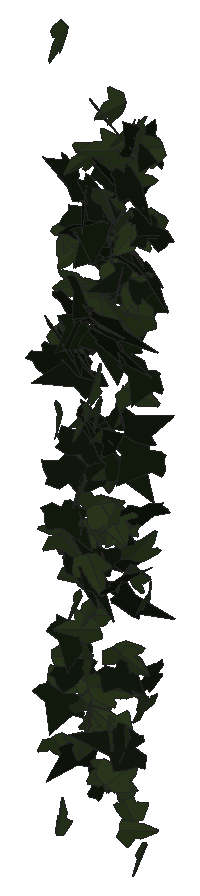
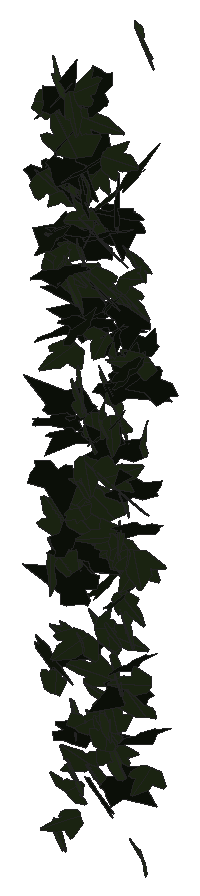
# SketchUp Ruby script. Lengths in inches.
U = 1.inch
M = Sketchup.active_model
def pt(a) = Geom::Point3d.new(a.map { |v| v * U })
def face(e, loops, mat)
  f = e.add_face(loops[0].map { |a| pt(a) })
  loops[1..].each { |l| e.add_face(l.map { |a| pt(a) }).erase! }
  f.material = f.back_material = mat if mat
  f
end
# faces: each face lists its corners as indices into pts; further lists are holes
def faces(e, pts, list, mat = nil) = list.each { |f| face(e, (f[0].is_a?(Array) ? f : [f]).map { |l| l.map { |i| pts[i] } }, mat) }
# xy, xz, yz: faces in a plane at the given z, y or x. An outline is a flat list of corners, or four numbers for a rectangle; further outlines are holes
def ring(l) = l.size == 4 ? [[l[0], l[1]], [l[2], l[1]], [l[2], l[3]], [l[0], l[3]]] : l.each_slice(2).to_a
def flat(e, list, mat, &to3) = list.each { |f| face(e, (f[0].is_a?(Array) ? f : [f]).map { |l| ring(l).map { |u, v| to3.(u, v) } }, mat) }
def xy(e, z, list, mat = nil) = flat(e, list, mat) { |x, y| [x, y, z] }
def xz(e, y, list, mat = nil) = flat(e, list, mat) { |x, z| [x, y, z] }
def yz(e, x, list, mat = nil) = flat(e, list, mat) { |y, z| [x, y, z] }
def lines(e, pts, list) = list.each { |a, b| e.add_line(pt(pts[a]), pt(pts[b])) }
# prism: a flat outline (further loops are holes) pulled along v
def prism(e, loops, v, mat = nil)
  f = face(e, loops, mat); d = Geom::Vector3d.new(v.map { |x| x * U })
  f.pushpull(f.normal.samedirection?(d) ? d.length : -d.length)
end
def box(e, o, s, mat = nil) = prism(e, [[o, [o[0] + s[0], o[1], o[2]], [o[0] + s[0], o[1] + s[1], o[2]], [o[0], o[1] + s[1], o[2]]]], [0, 0, s[2]], mat)
def at(x, y, z, deg = 0) = Geom::Transformation.translation(pt([x, y, z])) * Geom::Transformation.rotation(ORIGIN, Z_AXIS, deg.degrees)
def axes(o, x, y, z) = Geom::Transformation.new([*x, 0, *y, 0, *z, 0, *pt(o).to_a, 1])
def part(name) = M.definitions.add(name)
# library, detail: a bought-in or finely detailed component or shape, given as its bounding box
def library(name, o, s) = part(name).tap { |d| box(d.entities, o, s) }
def detail(e, o, s) = box(e.add_group.entities, o, s)
def put(e, d, t, mat = nil) = e.add_instance(d, t).tap { |i| i.material = mat if mat }
def group(e, t, mat = nil) = e.add_group.tap { |g| g.transformation = t; g.material = mat if mat }.entities
root = M.entities
M.materials.add("1026 AP 7946 SUNNY SIDE UP").color = [254, 231, 186]
M.materials.add("efeu1").color = [18, 25, 13]
M.materials.add("efeu2").color = [43, 57, 29]
c1 = part("ivyleaf_10")
p = [[0,0.5,-0.03],[-0.0625,2.02,-0.43],[-0.19,2.01,-0.46],[-0.54,1.05,-0.29],[-0.52,0.625,-0.18],[-0.83,0.76,-0.28],
  [-1.16,0.64,-0.33],[-1.15,0.33,-0.24],[-0.77,-0.39,0.02],[-0.3,-0.51,0.16],[0.04,-0.48,0.23],[-0.02,2.01,-0.4375],
  [-0.06,2.01,-0.43],[0.04,-0.49,0.23],[0.67,-0.49,0.14],[1.38,0.36,-0.2],[1.375,0.51,-0.24],[0.81,0.65,-0.19],
  [0.62,0.59,-0.15],[0.6,1.09,-0.28],[0.5,1.23,-0.31]]
faces(c1.entities,p,[[0,1,2,3,4,5,6,7,8,9,10],[11,12,0,13,14,15,16,17,18,19,20]],"efeu2")
c2 = part("ivyleaf_9")
p = [[1.54,2.16,1.25],[1.36,2.04,1.19],[-0.21,0.99,0.68],[-0.71,1.11,0.82],[-0.85,0.86,0.67],[-0.8,0.17,0.21],
  [-0.9,-0.01,0.1],[-0.67,-0.16,-0.02],[-0.08,-0.08,-0.05],[-0.03,-0.6,-0.4],[0.65,-0.88,-0.66],[0.83,-0.6,-0.49],
  [1.29,-0.42,-0.43],[1.8125,-0.07,-0.26],[1.21,0.44,0.15]]
faces(c2.entities,p,[[0,1,2,3,4,5,6,7,8,9,10,11,12,13,14]],"efeu1")
put(root,c1,axes([111.04,211.59,258.61],[0.30252,-0.15607,0.01746],[0.00318,-0.02574,-0.25464],[0.24698,0.1915,-0.01812]),"1026 AP 7946 SUNNY SIDE UP")
put(root,c2,axes([110.8125,211.57,261.93],[0.31359,-0.0983,0.17351],[0.21726,-0.0999,-0.22844],[0.21747,0.24155,-0.02198]),"1026 AP 7946 SUNNY SIDE UP")
put(root,c2,axes([110.88,211.54,262.32],[0.30214,-0.05478,0.18215],[0.25651,-0.07125,-0.20544],[0.13851,0.25143,-0.01687]),"1026 AP 7946 SUNNY SIDE UP")
put(root,c2,axes([109.72,211.71,261.66],[0.07676,-0.16825,0.19826],[0.10699,-0.18132,-0.18125],[0.38863,0.08315,0.01074]),"1026 AP 7946 SUNNY SIDE UP")
put(root,c1,axes([110.43,211.59,260.29],[0.19919,-0.26197,-0.00928],[-0.01864,0.00261,-0.2996],[0.41167,0.12687,-0.00908]),"1026 AP 7946 SUNNY SIDE UP")
put(root,c1,axes([109.73,211.73,259.9375],[-0.01994,0.01186,0.27147],[0.24473,-0.21258,0.01633],[0.33474,0.15613,0.00423]),"1026 AP 7946 SUNNY SIDE UP")
put(root,c1,axes([110.51,211.61,257.3],[0.33232,0.00269,0.16449],[0.24963,-0.03192,-0.21614],[0.0269,0.26294,-0.02637]),"1026 AP 7946 SUNNY SIDE UP")
put(root,c1,axes([111.43,211.56,262.43],[-0.38192,0.01159,-0.18672],[-0.28045,0.04243,0.24918],[0.0544,0.30011,-0.02623]),"1026 AP 7946 SUNNY SIDE UP")
put(root,c1,axes([110.82,211.48,254.89],[-0.07067,-0.00583,0.26294],[0.34009,0.13688,0.04325],[-0.21338,0.2201,-0.01814]),"1026 AP 7946 SUNNY SIDE UP")
put(root,c1,axes([110.96,211.53,258.52],[0.32672,0.13462,0.13671],[0.18289,0.06295,-0.25451],[-0.23322,0.23795,-0.00807]),"1026 AP 7946 SUNNY SIDE UP")
put(root,c1,axes([111.46,211.49,254.04],[0.10164,-0.19933,-0.15373],[-0.05275,0.14462,-0.21476],[0.38688,0.07208,0.01111]),"1026 AP 7946 SUNNY SIDE UP")
put(root,c2,axes([110.3125,211.77,261.92],[-0.2114,-0.15335,0.13328],[-0.09465,-0.11882,-0.20882],[0.30187,-0.14464,0.02786]),"1026 AP 7946 SUNNY SIDE UP")
put(root,c2,axes([110.28,211.83,262.58],[-0.06592,-0.16503,0.247],[-0.05104,-0.23902,-0.17606],[0.45604,-0.05061,0.016]),"1026 AP 7946 SUNNY SIDE UP")
put(root,c1,axes([110.35,211.625,258.81],[0.14496,-0.22878,-0.01015],[-0.01654,0.00498,-0.25394],[0.3596,0.09245,-0.00759]),"1026 AP 7946 SUNNY SIDE UP")
put(root,c2,axes([109.92,211.6,258.18],[0.01376,-0.19547,-0.15045],[0.09737,0.14204,-0.19267],[0.37004,-0.03011,0.05629]),"1026 AP 7946 SUNNY SIDE UP")
put(root,c2,axes([110.08,211.77,264.91],[0.11972,-0.28684,-0.03214],[0.04752,-0.02247,0.30466],[-0.45093,-0.07852,0.02358]),"1026 AP 7946 SUNNY SIDE UP")
put(root,c1,axes([110.48,211.7,255.89],[-0.09368,-0.01887,0.24048],[-0.28086,-0.15228,-0.06051],[0.23841,-0.18681,0.02321]),"1026 AP 7946 SUNNY SIDE UP")
put(root,c2,axes([111.2,211.54,255.375],[0.00797,-0.13008,-0.21277],[0.01462,0.20579,-0.13257],[0.38253,-0.00515,0.0095]),"1026 AP 7946 SUNNY SIDE UP")
put(root,c1,axes([109.84,211.67,267.88],[0.26284,-0.25087,0.012],[-0.00612,-0.01829,-0.31036],[0.39496,0.16667,-0.01279]),"1026 AP 7946 SUNNY SIDE UP")
put(root,c1,axes([111.1875,211.7,257.14],[0.03813,-0.20313,-0.09742],[0.06358,-0.08842,0.20839],[-0.34575,-0.03866,0.02758]),"1026 AP 7946 SUNNY SIDE UP")
put(root,c2,axes([111.21,211.41,257.17],[-0.05601,0.19,-0.1722],[-0.03869,0.1665,0.20005],[0.39716,0.04302,-0.0048]),"1026 AP 7946 SUNNY SIDE UP")
put(root,c2,axes([111.38,211.77,253.75],[-0.15816,-0.15471,-0.22356],[-0.19168,-0.17849,0.18903],[-0.37139,0.15801,-0.00236]),"1026 AP 7946 SUNNY SIDE UP")
put(root,c2,axes([110.59,211.73,259.74],[-0.09981,-0.00293,0.27434],[0.25802,-0.21606,0.03657],[0.32984,0.16813,0.0544]),"1026 AP 7946 SUNNY SIDE UP")
put(root,c1,axes([110.45,211.6875,253.625],[-0.23115,-0.16581,0.07334],[-0.05359,-0.06589,-0.22797],[0.27923,-0.14991,0.01696]),"1026 AP 7946 SUNNY SIDE UP")
put(root,c1,axes([109.74,211.59,253.39],[-0.18971,-0.14311,-0.11144],[0.13133,0.06946,-0.19167],[0.24877,-0.1458,0.0162]),"1026 AP 7946 SUNNY SIDE UP")
put(root,c2,axes([111.46,211.82,263.36],[-0.01003,-0.07,-0.263],[-0.0769,-0.25025,0.0706],[-0.40846,0.04883,-0.00684]),"1026 AP 7946 SUNNY SIDE UP")
put(root,c1,axes([111.11,211.77,265.89],[-0.10047,-0.0406,0.28246],[-0.32021,-0.18435,-0.07803],[0.29619,-0.21307,0.01146]),"1026 AP 7946 SUNNY SIDE UP")
put(root,c2,axes([109.77,211.83,254.22],[-0.17093,-0.23263,0.05842],[-0.0224,-0.05733,-0.26461],[0.37633,-0.10907,0.01078]),"1026 AP 7946 SUNNY SIDE UP")
put(root,c1,axes([111.22,211.74,255.57],[-0.06018,-0.01159,-0.24218],[0.30076,-0.14021,-0.02579],[-0.21549,-0.19246,0.03164]),"1026 AP 7946 SUNNY SIDE UP")
put(root,c1,axes([111.1,211.53,253.09],[0.25615,0.08611,-0.18998],[0.22602,0.11942,0.18846],[0.22755,-0.21556,0.02666]),"1026 AP 7946 SUNNY SIDE UP")
put(root,c1,axes([111.26,211.73,264.59],[0.06491,-0.26607,0.03363],[0.00067,-0.03449,-0.27754],[0.4218,0.041,-0.00474]),"1026 AP 7946 SUNNY SIDE UP")
put(root,c2,axes([111.62,211.85,261.5],[-0.14273,-0.21925,0.09189],[-0.02525,-0.09094,-0.24423],[0.37207,-0.09028,0.01868]),"1026 AP 7946 SUNNY SIDE UP")
put(root,c2,axes([110.45,211.73,256.98],[0.18394,-0.23826,-0.02048],[-0.02931,0.01147,-0.27311],[0.37463,0.11788,-0.01131]),"1026 AP 7946 SUNNY SIDE UP")
put(root,c1,axes([110.81,211.69,264.87],[-0.34515,0.07392,-0.09062],[0.10977,-0.06595,-0.23583],[-0.14412,-0.22725,0.03739]),"1026 AP 7946 SUNNY SIDE UP")
put(root,c2,axes([110.23,211.88,261.85],[0.03763,-0.09908,-0.23194],[0.18695,-0.19273,0.09952],[-0.33767,-0.11774,0.02925]),"1026 AP 7946 SUNNY SIDE UP")
put(root,c1,axes([111.42,211.84,266.28],[0.08577,-0.18091,-0.2197],[0.13687,-0.1944,0.19262],[-0.41659,-0.10111,0.01805]),"1026 AP 7946 SUNNY SIDE UP")
put(root,c1,axes([111.4,211.79,264.29],[0.21146,0.13552,-0.16404],[-0.14874,-0.13043,-0.19648],[-0.29425,0.16332,-0.01857]),"1026 AP 7946 SUNNY SIDE UP")
put(root,c1,axes([109.84,211.65,254.59],[0.32946,-0.00035,-0.08441],[0.12818,0.02364,0.21478],[0.01302,-0.22373,0.0215]),"1026 AP 7946 SUNNY SIDE UP")
put(root,c1,axes([111.59,211.79,251.71],[0.15704,-0.1968,0.08996],[0.05404,-0.0817,-0.22775],[0.33493,0.10546,-0.00543]),"1026 AP 7946 SUNNY SIDE UP")
put(root,c2,axes([111.29,211.69,265.47],[0.18631,-0.24542,-0.14088],[-0.11516,0.11473,-0.27969],[0.42538,0.13855,-0.01402]),"1026 AP 7946 SUNNY SIDE UP")
put(root,c2,axes([110.43,211.79,264.25],[-0.19814,-0.22234,-0.08522],[0.07164,0.06779,-0.26282],[0.36538,-0.13387,0.00532]),"1026 AP 7946 SUNNY SIDE UP")
put(root,c2,axes([109.95,211.86,255.58],[-0.09419,-0.24462,0.053],[-0.01081,-0.0527,-0.25969],[0.39336,-0.06002,0.00555]),"1026 AP 7946 SUNNY SIDE UP")
put(root,c1,axes([110.16,211.71,256.35],[0.12527,-0.23551,-0.04232],[-0.02974,0.03554,-0.25584],[0.37438,0.08163,-0.00616]),"1026 AP 7946 SUNNY SIDE UP")
put(root,c1,axes([110.83,211.6875,253.08],[0.2315,-0.13655,-0.12404],[-0.16545,0.06132,-0.20517],[0.23262,0.17952,-0.02248]),"1026 AP 7946 SUNNY SIDE UP")
put(root,c1,axes([111.44,211.65,252.48],[0.30643,-0.0041,0.13761],[-0.20804,0.02767,0.19985],[-0.02989,-0.23465,0.01977]),"1026 AP 7946 SUNNY SIDE UP")
put(root,c2,axes([110.57,211.89,263.79],[-0.24726,-0.16841,0.09756],[-0.04563,-0.10133,-0.23353],[0.3011,-0.15365,0.04472]),"1026 AP 7946 SUNNY SIDE UP")
put(root,c2,axes([110.32,211.6,264.14],[0.10249,0.23385,-0.03723],[-0.00687,-0.03766,-0.25024],[-0.37233,0.06507,-0.00563]),"1026 AP 7946 SUNNY SIDE UP")
put(root,c2,axes([110.61,211.77,266.52],[0.34266,-0.19567,0.07654],[0.06497,-0.06655,-0.30132],[0.32327,0.22079,-0.02057]),"1026 AP 7946 SUNNY SIDE UP")
put(root,c1,axes([109.85,211.62,251.64],[0.25098,-0.13366,0.13633],[-0.13923,0.10085,0.21432],[-0.26187,-0.18171,0.0167]),"1026 AP 7946 SUNNY SIDE UP")
put(root,c1,axes([111.76,211.7,262.74],[-0.09806,0.0313,0.25254],[-0.38647,-0.03248,-0.06037],[0.03783,-0.25068,0.03784]),"1026 AP 7946 SUNNY SIDE UP")
put(root,c1,axes([111.04,211.82,263.29],[0.18792,-0.1703,0.13009],[0.12082,-0.1015,-0.21489],[0.31167,0.14203,0.00486]),"1026 AP 7946 SUNNY SIDE UP")
put(root,c1,axes([111.6,211.84,254.58],[-0.0346,-0.21421,-0.14712],[-0.02936,-0.1404,0.22099],[-0.40269,0.02864,-0.00347]),"1026 AP 7946 SUNNY SIDE UP")
put(root,c1,axes([110.55,211.78,254.03],[0.27196,-0.02252,0.19552],[0.28777,-0.05486,-0.17872],[0.08732,0.25095,-0.01998]),"1026 AP 7946 SUNNY SIDE UP")
put(root,c2,axes([109.51,211.625,261.23],[0.03966,0.00803,-0.26584],[0.2488,0.20446,0.02368],[0.32087,-0.15952,0.0145]),"1026 AP 7946 SUNNY SIDE UP")
put(root,c2,axes([110.15,211.85,253.27],[-0.04611,0.09563,-0.26568],[0.08453,-0.25292,-0.10418],[-0.42497,-0.06068,0.0081]),"1026 AP 7946 SUNNY SIDE UP")
put(root,c1,axes([110.29,211.71,257.76],[-0.34124,-0.08445,-0.02154],[0.04149,-0.0117,-0.23905],[0.13017,-0.21766,0.01974]),"1026 AP 7946 SUNNY SIDE UP")
put(root,c2,axes([111.6,211.9,259.84],[-0.30443,-0.18822,0.05832],[-0.03808,-0.05751,-0.27743],[0.30719,-0.19366,0.0234]),"1026 AP 7946 SUNNY SIDE UP")
put(root,c1,axes([110.76,211.65,262.76],[0.12597,-0.06737,-0.26799],[-0.34837,0.13635,-0.10603],[0.23809,0.23516,-0.01335]),"1026 AP 7946 SUNNY SIDE UP")
put(root,c1,axes([110.42,211.68,254.58],[0.21207,-0.02835,-0.17613],[0.27226,0.02239,0.13715],[0.00039,-0.21648,0.03594]),"1026 AP 7946 SUNNY SIDE UP")
put(root,c2,axes([110.19,211.88,264.2],[0.0228,0.06409,0.278],[-0.08496,-0.26401,0.06613],[0.42719,-0.05593,-0.00169]),"1026 AP 7946 SUNNY SIDE UP")
put(root,c1,axes([111.04,211.61,263.32],[0.10254,0.00601,-0.27286],[0.37624,0.11584,0.06407],[0.17895,-0.24699,0.02164]),"1026 AP 7946 SUNNY SIDE UP")
put(root,c2,axes([111.24,211.71,259.6],[-0.00485,-0.18907,-0.17933],[0.07199,0.16983,-0.19105],[0.39649,-0.03315,0.0325]),"1026 AP 7946 SUNNY SIDE UP")
put(root,c1,axes([110.32,211.76,254.22],[-0.14333,-0.20443,-0.00993],[-0.00581,-0.00764,0.23055],[-0.32167,0.09123,0.00026]),"1026 AP 7946 SUNNY SIDE UP")
put(root,c2,axes([110.65,211.77,265.35],[0.33046,-0.13118,0.10543],[0.11864,-0.07315,-0.25478],[0.23398,0.22236,-0.01972]),"1026 AP 7946 SUNNY SIDE UP")
put(root,c2,axes([110.88,211.81,261.97],[-0.20331,-0.2129,-0.11673],[0.11914,0.08476,-0.25536],[0.35908,-0.14866,0.01863]),"1026 AP 7946 SUNNY SIDE UP")
put(root,c2,axes([110.24,211.89,261.01],[-0.03357,-0.05235,-0.27746],[-0.12071,-0.25791,0.05646],[-0.41371,0.0795,0.00604]),"1026 AP 7946 SUNNY SIDE UP")
put(root,c1,axes([110.47,211.61,255.3],[0.12164,-0.13196,-0.22023],[-0.13558,0.19531,-0.15576],[0.36996,0.11497,0.01532]),"1026 AP 7946 SUNNY SIDE UP")
put(root,c1,axes([111.01,211.8,253.98],[0.15395,0.16213,0.15875],[-0.14515,-0.12283,0.194],[0.31927,-0.13402,0.01165]),"1026 AP 7946 SUNNY SIDE UP")
put(root,c1,axes([111.43,211.63,261.14],[-0.12914,-0.15658,-0.21561],[0.24134,0.14755,-0.17566],[0.33128,-0.16853,0.04392]),"1026 AP 7946 SUNNY SIDE UP")
put(root,c2,axes([110.92,211.84,263.73],[-0.29145,-0.18164,-0.12187],[0.15205,0.0685,-0.26637],[0.30406,-0.20836,0.01639]),"1026 AP 7946 SUNNY SIDE UP")
put(root,c2,axes([110.85,211.77,257.26],[0.06379,0.00681,0.24596],[-0.35962,0.0708,0.03837],[-0.10808,-0.23155,0.01749]),"1026 AP 7946 SUNNY SIDE UP")
put(root,c2,axes([110.05,211.68,262.45],[0.34158,0.01201,-0.17462],[-0.26355,-0.03078,-0.22363],[-0.0446,0.27385,-0.01585]),"1026 AP 7946 SUNNY SIDE UP")
put(root,c2,axes([110.02,211.65,258.78],[-0.27279,-0.06754,0.20529],[0.28056,0.09059,0.19182],[-0.17642,0.2485,-0.01238]),"1026 AP 7946 SUNNY SIDE UP")
put(root,c1,axes([110.5,211.74,258.36],[-0.29114,-0.01549,0.21155],[0.31203,0.0608,0.18933],[-0.08704,0.2698,-0.02886]),"1026 AP 7946 SUNNY SIDE UP")
put(root,c1,axes([110.36,211.92,254.15],[0.01701,-0.14875,-0.20932],[0.02381,-0.20178,0.15246],[-0.39417,-0.01861,0.00018]),"1026 AP 7946 SUNNY SIDE UP")
put(root,c1,axes([111.4,211.67,263.15],[0.03368,0.23003,0.09715],[0.02288,0.09202,-0.23739],[-0.38947,0.0253,-0.00555]),"1026 AP 7946 SUNNY SIDE UP")
put(root,c1,axes([110.16,211.82,253.4],[0.09342,-0.2355,-0.06153],[0.07133,-0.04827,0.24785],[-0.37479,-0.06789,0.03183]),"1026 AP 7946 SUNNY SIDE UP")
put(root,c1,axes([111.02,211.82,258.2],[0.2172,0.15288,-0.0913],[-0.084,-0.07224,-0.21253],[-0.26558,0.14788,-0.00745]),"1026 AP 7946 SUNNY SIDE UP")
put(root,c2,axes([110.3,211.67,259.46],[-0.2107,-0.00172,0.24745],[0.37529,0.03015,0.13756],[-0.0427,0.2734,-0.01199]),"1026 AP 7946 SUNNY SIDE UP")
put(root,c1,axes([110.26,211.96,265.43],[-0.03555,-0.12358,0.24543],[-0.02042,-0.239,-0.13001],[0.42249,-0.02195,0.01437]),"1026 AP 7946 SUNNY SIDE UP")
put(root,c1,axes([109.85,211.625,255.13],[-0.02375,-0.00694,0.23098],[0.14615,0.20436,0.01416],[-0.32107,0.09354,-0.01064]),"1026 AP 7946 SUNNY SIDE UP")
put(root,c2,axes([110.6875,211.72,263.58],[0.1523,0.04321,-0.22496],[0.26766,0.1395,0.10691],[0.22614,-0.1942,0.02497]),"1026 AP 7946 SUNNY SIDE UP")
put(root,c1,axes([109.87,211.8,257.66],[-0.33492,-0.15001,0.04564],[-0.03482,-0.04661,-0.26742],[0.24386,-0.21268,0.0245]),"1026 AP 7946 SUNNY SIDE UP")
put(root,c2,axes([111.86,211.79,264.58],[0.02122,0.01963,-0.25707],[-0.32409,-0.14111,-0.02374],[-0.22362,0.20638,0.01]),"1026 AP 7946 SUNNY SIDE UP")
put(root,c2,axes([110.05,211.65,254.96],[0.02046,-0.06204,-0.25992],[0.04692,0.25095,-0.06061],[0.4053,-0.02592,0.02014]),"1026 AP 7946 SUNNY SIDE UP")
put(root,c1,axes([110.51,211.71,260.69],[0.23621,-0.19596,0.10787],[-0.08361,0.09239,0.25456],[-0.34005,-0.15883,0.01234]),"1026 AP 7946 SUNNY SIDE UP")
put(root,c2,axes([111.43,211.91,266.03],[0.12073,0.10502,0.26504],[-0.27633,-0.18761,0.13214],[0.33734,-0.19126,0.01339]),"1026 AP 7946 SUNNY SIDE UP")
put(root,c1,axes([110.98,211.74,257.91],[-0.24096,-0.09859,0.14597],[0.1652,0.098,0.18714],[-0.21627,0.1847,-0.01969]),"1026 AP 7946 SUNNY SIDE UP")
put(root,c1,axes([110.24,211.8,257.77],[-0.27444,0.06165,-0.142],[0.19108,-0.0686,-0.19004],[-0.14178,-0.21179,0.01875]),"1026 AP 7946 SUNNY SIDE UP")
put(root,c1,axes([111.48,211.75,257.75],[-0.13278,-0.23877,0.09864],[0.05979,0.08953,0.26137],[-0.40086,0.09244,0.00631]),"1026 AP 7946 SUNNY SIDE UP")
put(root,c2,axes([110.36,211.97,260.06],[0.02662,-0.24668,0.1171],[0.00731,-0.11502,-0.25538],[0.42794,0.01731,-0.00292]),"1026 AP 7946 SUNNY SIDE UP")
put(root,c2,axes([111,211.82,256.68],[0.22697,-0.05669,0.24977],[0.33452,-0.11823,-0.15944],[0.20435,0.2565,-0.0164]),"1026 AP 7946 SUNNY SIDE UP")
put(root,c1,axes([110.78,211.79,260.02],[-0.03862,-0.25219,-0.03739],[0.01662,0.03398,-0.26073],[0.39997,-0.02577,0.00722]),"1026 AP 7946 SUNNY SIDE UP")
put(root,c2,axes([110.72,211.87,262.77],[-0.38008,0.06393,-0.07498],[0.10031,-0.04346,-0.25658],[-0.1152,-0.24878,0.02396]),"1026 AP 7946 SUNNY SIDE UP")
put(root,c1,axes([110.14,211.78,262.79],[0.24196,-0.05273,-0.18149],[-0.2552,0.06822,-0.16697],[0.13498,0.2235,0.00965]),"1026 AP 7946 SUNNY SIDE UP")
put(root,c1,axes([109.84,211.73,257.52],[-0.23638,-0.17674,-0.13348],[0.14781,0.08858,-0.23817],[0.31025,-0.17686,0.01177]),"1026 AP 7946 SUNNY SIDE UP")
put(root,c1,axes([111.18,211.87,262.57],[0.12587,-0.22498,0.04111],[0.00949,-0.04154,-0.24611],[0.35952,0.07986,-0.0079]),"1026 AP 7946 SUNNY SIDE UP")
put(root,c2,axes([109.87,211.97,261.46],[0.11128,-0.19028,0.16619],[0.08758,-0.15256,-0.21004],[0.38349,0.09006,-0.00026]),"1026 AP 7946 SUNNY SIDE UP")
put(root,c1,axes([110.87,211.89,264.64],[-0.20721,0.14532,-0.15049],[0.07303,-0.14895,-0.19558],[-0.3166,-0.12946,0.05338]),"1026 AP 7946 SUNNY SIDE UP")
put(root,c1,axes([111.125,211.79,252.79],[0.2668,-0.17603,0.01267],[0.00578,0.02197,0.25133],[-0.27751,-0.16877,0.01742]),"1026 AP 7946 SUNNY SIDE UP")
put(root,c1,axes([110.08,211.9375,257.8125],[-0.11607,0.11354,0.22332],[0.22819,-0.16117,0.13734],[0.3087,0.16182,-0.01756]),"1026 AP 7946 SUNNY SIDE UP")
put(root,c2,axes([111.6,211.74,258.73],[0.12676,0.23036,-0.09136],[-0.0342,-0.08768,-0.2518],[-0.38736,0.08312,-0.00766]),"1026 AP 7946 SUNNY SIDE UP")
put(root,c1,axes([110.83,212.03,266.6],[-0.02371,-0.00215,0.29125],[0.07193,-0.27942,-0.00131],[0.43871,0.0457,0.01595]),"1026 AP 7946 SUNNY SIDE UP")
put(root,c1,axes([110.42,211.91,253.91],[-0.10393,-0.21527,-0.09811],[-0.06172,-0.08617,0.23119],[-0.36417,0.07604,-0.01118]),"1026 AP 7946 SUNNY SIDE UP")
put(root,c1,axes([109.68,211.82,261.58],[-0.12553,-0.06304,-0.2204],[0.34992,-0.01418,-0.08146],[0.01297,-0.22757,0.06469]),"1026 AP 7946 SUNNY SIDE UP")
put(root,c2,axes([110.42,211.99,264.51],[0.04596,-0.28997,-0.03755],[0.01313,-0.03413,0.3],[-0.45903,-0.03001,0.00482]),"1026 AP 7946 SUNNY SIDE UP")
put(root,c2,axes([111.24,211.88,257.44],[0.12699,0.15777,0.17515],[-0.19955,-0.11953,0.17661],[0.30404,-0.14435,0.04276]),"1026 AP 7946 SUNNY SIDE UP")
put(root,c1,axes([111.08,211.76,255.62],[-0.25483,-0.12086,-0.17908],[0.24122,0.08258,-0.20683],[0.22814,-0.22232,0.01866]),"1026 AP 7946 SUNNY SIDE UP")
put(root,c2,axes([110.85,212,264.6],[-0.11641,-0.01504,-0.24263],[0.30448,-0.14483,-0.05404],[-0.2119,-0.19984,0.05564]),"1026 AP 7946 SUNNY SIDE UP")
put(root,c1,axes([110.4,212.03,256.2],[0.03616,-0.09,0.23968],[0.08602,-0.22666,-0.09702],[0.38346,0.05933,-0.00083]),"1026 AP 7946 SUNNY SIDE UP")
put(root,c1,axes([111.72,211.96,266.06],[0.0748,0.0259,-0.25257],[-0.3295,-0.12756,-0.05648],[-0.20463,0.21487,-0.00137]),"1026 AP 7946 SUNNY SIDE UP")
put(root,c1,axes([110.25,211.93,255.98],[0.16033,-0.09745,-0.22604],[0.27468,-0.13254,0.14386],[-0.2578,-0.20182,0.01271]),"1026 AP 7946 SUNNY SIDE UP")
put(root,c2,axes([111.52,212.08,266.07],[-0.05536,-0.20776,0.19798],[-0.03828,-0.19191,-0.21812],[0.44463,-0.04239,0.00587]),"1026 AP 7946 SUNNY SIDE UP")
put(root,c1,axes([111.2,211.67,260.625],[-0.08188,0.09874,0.28527],[-0.31927,0.19051,-0.10843],[-0.33315,-0.20684,0.0338]),"1026 AP 7946 SUNNY SIDE UP")
put(root,c2,axes([110.89,212.07,261.84],[-0.00827,-0.18253,0.22078],[0.02459,-0.21524,-0.18882],[0.4432,0.00854,0.01459]),"1026 AP 7946 SUNNY SIDE UP")
put(root,c1,axes([110.4,211.71,257.87],[0.00326,0.03837,0.25239],[0.18671,0.21469,-0.03445],[-0.34193,0.11759,-0.01641]),"1026 AP 7946 SUNNY SIDE UP")
put(root,c1,axes([110.32,211.85,260.15],[-0.07968,-0.24595,-0.04733],[0.02096,0.04273,-0.25841],[0.39247,-0.05222,0.00419]),"1026 AP 7946 SUNNY SIDE UP")
put(root,c1,axes([110.4,212.02,260.28],[0.10446,-0.11004,0.20367],[0.16953,-0.16649,-0.13335],[0.31375,0.1266,0.00425]),"1026 AP 7946 SUNNY SIDE UP")
put(root,c1,axes([110.67,211.98,264],[-0.08417,0.19564,-0.18762],[0.069,-0.17793,-0.20996],[-0.41579,-0.06913,0.00314]),"1026 AP 7946 SUNNY SIDE UP")
put(root,c2,axes([111.67,211.77,264.32],[-0.08213,0.12906,0.21509],[-0.24881,0.14454,-0.13245],[-0.29377,-0.1585,0.05204]),"1026 AP 7946 SUNNY SIDE UP")
put(root,c1,axes([110.08,211.85,256.81],[-0.2042,0.02495,0.18085],[-0.27821,-0.00693,-0.13397],[-0.01452,-0.21814,0.02365]),"1026 AP 7946 SUNNY SIDE UP")
put(root,c1,axes([109.79,211.93,263.67],[0.33116,-0.11483,-0.00415],[-0.02061,-0.01702,-0.24625],[0.17945,0.20995,-0.02062]),"1026 AP 7946 SUNNY SIDE UP")
put(root,c1,axes([111.68,211.8,256.96],[0.02946,-0.22163,-0.15341],[-0.0113,0.14755,-0.22823],[0.4186,0.01958,0.00463]),"1026 AP 7946 SUNNY SIDE UP")
put(root,c2,axes([110.73,211.73,252.68],[-0.03166,0.10811,0.22383],[-0.12102,0.20327,-0.11067],[-0.36098,-0.07763,0.01747]),"1026 AP 7946 SUNNY SIDE UP")
put(root,c1,axes([111.65,212.03,264.5625],[-0.18234,-0.16178,0.18166],[-0.04671,-0.18567,-0.19569],[0.37445,-0.10194,0.06405]),"1026 AP 7946 SUNNY SIDE UP")
put(root,c2,axes([109.9375,211.97,257.01],[0.14629,-0.26034,-0.00907],[-0.01865,0.00353,-0.28461],[0.4091,0.09326,-0.00973]),"1026 AP 7946 SUNNY SIDE UP")
put(root,c1,axes([110.94,211.91,260.3],[0.13093,-0.2296,-0.02005],[0.02198,-0.01423,0.25137],[-0.36148,-0.08403,0.00803]),"1026 AP 7946 SUNNY SIDE UP")
put(root,c1,axes([110.84,211.91,259.21],[-0.09796,-0.26453,-0.00717],[0.01758,0.00297,-0.27976],[0.41566,-0.06247,0.01014]),"1026 AP 7946 SUNNY SIDE UP")
put(root,c2,axes([110.59,211.85,259.06],[-0.29262,0.17326,0.11698],[-0.16491,0.05132,-0.25969],[-0.27992,-0.21135,0.03071]),"1026 AP 7946 SUNNY SIDE UP")
put(root,c2,axes([111.19,211.84,260.15],[-0.06075,0.02792,0.26586],[0.39877,-0.0508,0.04451],[0.08582,0.25579,-0.01861]),"1026 AP 7946 SUNNY SIDE UP")
put(root,c2,axes([111.41,212.0625,263.52],[0.1321,-0.24004,0.14061],[0.07538,-0.12927,-0.26275],[0.42868,0.0967,0.00287]),"1026 AP 7946 SUNNY SIDE UP")
put(root,c1,axes([110.29,211.98,259.21],[-0.19973,-0.06078,-0.22232],[-0.33006,-0.05379,0.1428],[-0.12238,0.24426,-0.02229]),"1026 AP 7946 SUNNY SIDE UP")
put(root,c1,axes([111.15,211.9,265.33],[-0.40911,-0.1178,0.10849],[0.13711,0.06368,0.29383],[-0.20804,0.27362,-0.01969]),"1026 AP 7946 SUNNY SIDE UP")
put(root,c1,axes([109.83,212.08,263.27],[-0.11826,-0.07365,0.22064],[0.05506,-0.22713,-0.06899],[0.35246,0.01077,0.08481]),"1026 AP 7946 SUNNY SIDE UP")
put(root,c1,axes([111.25,211.76,252.04],[-0.01559,-0.07003,-0.2421],[0.24368,0.17998,-0.06104],[0.29804,-0.15081,0.03724]),"1026 AP 7946 SUNNY SIDE UP")
put(root,c2,axes([110.76,212.08,265.11],[-0.0487,-0.27171,0.06379],[-0.00506,-0.0635,-0.28207],[0.43871,-0.0309,0.00383]),"1026 AP 7946 SUNNY SIDE UP")
put(root,c2,axes([111.79,211.95,255.32],[-0.28895,0.14024,-0.09021],[0.09087,-0.06943,-0.23776],[-0.24428,-0.19171,0.01825]),"1026 AP 7946 SUNNY SIDE UP")
put(root,c1,axes([111.18,211.98,257.12],[-0.19826,0.0316,0.21243],[0.31326,-0.0525,0.1336],[0.09633,0.23577,0.00275]),"1026 AP 7946 SUNNY SIDE UP")
put(root,c1,axes([111.15,211.91,266.23],[0.00558,-0.2747,-0.05051],[-0.00347,0.04744,-0.28273],[0.43832,0.00387,-0.00159]),"1026 AP 7946 SUNNY SIDE UP")
put(root,c2,axes([111.26,211.96,265.04],[-0.09984,0.18501,-0.17905],[0.03059,-0.17616,-0.20033],[-0.39911,-0.05978,0.02944]),"1026 AP 7946 SUNNY SIDE UP")
put(root,c2,axes([109.73,212.1,261.45],[0.06203,-0.23091,0.1424],[0.0237,-0.13891,-0.24202],[0.42356,0.04159,-0.00731]),"1026 AP 7946 SUNNY SIDE UP")
put(root,c2,axes([110.77,211.82,263.74],[-0.18902,0.1596,0.14862],[-0.1522,0.1063,-0.20492],[-0.30104,-0.15396,0.01028]),"1026 AP 7946 SUNNY SIDE UP")
put(root,c1,axes([110.48,211.92,261.82],[-0.33157,0.07912,-0.04957],[0.05592,-0.0425,-0.23064],[-0.13485,-0.21218,0.02625]),"1026 AP 7946 SUNNY SIDE UP")
put(root,c1,axes([110.68,211.9375,264.08],[0.19742,0.01055,0.21656],[0.32776,0.02718,-0.12954],[-0.04518,0.24329,0.00653]),"1026 AP 7946 SUNNY SIDE UP")
put(root,c2,axes([111.34,212.0625,262.91],[-0.14338,-0.26477,-0.03793],[0.03583,0.02947,-0.28806],[0.41849,-0.09324,0.01167]),"1026 AP 7946 SUNNY SIDE UP")
